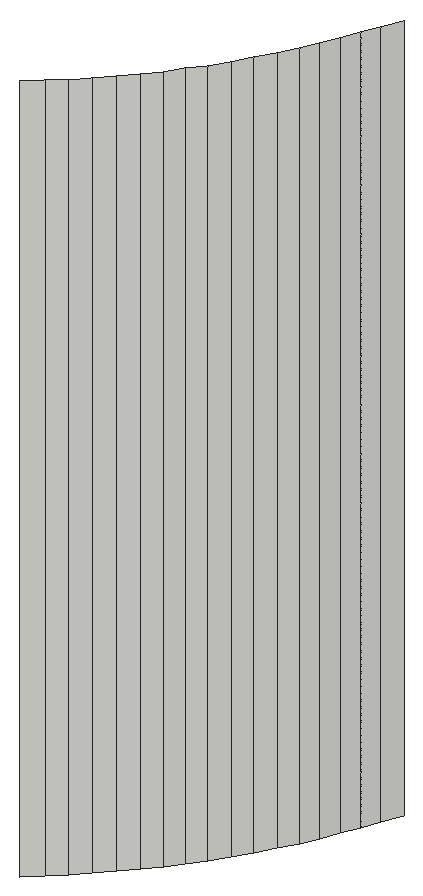
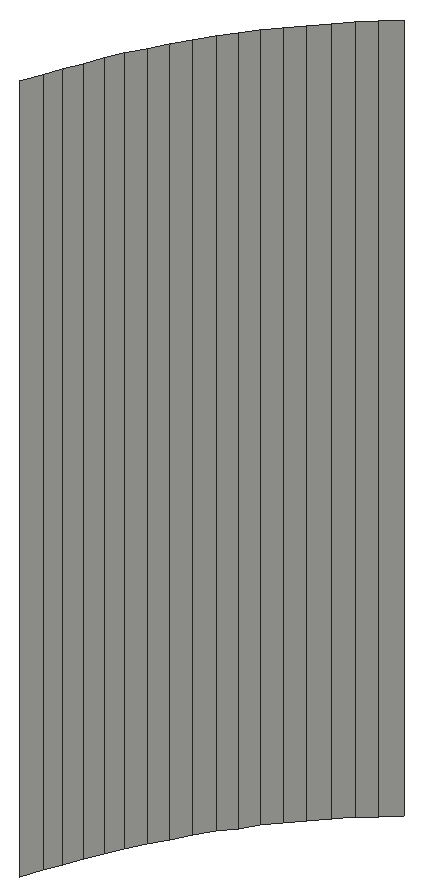
# SketchUp Ruby script. Lengths in inches.
U = 1.inch
M = Sketchup.active_model
def pt(a) = Geom::Point3d.new(a.map { |v| v * U })
def face(e, loops, mat)
  f = e.add_face(loops[0].map { |a| pt(a) })
  loops[1..].each { |l| e.add_face(l.map { |a| pt(a) }).erase! }
  f.material = f.back_material = mat if mat
  f
end
# faces: each face lists its corners as indices into pts; further lists are holes
def faces(e, pts, list, mat = nil) = list.each { |f| face(e, (f[0].is_a?(Array) ? f : [f]).map { |l| l.map { |i| pts[i] } }, mat) }
# xy, xz, yz: faces in a plane at the given z, y or x. An outline is a flat list of corners, or four numbers for a rectangle; further outlines are holes
def ring(l) = l.size == 4 ? [[l[0], l[1]], [l[2], l[1]], [l[2], l[3]], [l[0], l[3]]] : l.each_slice(2).to_a
def flat(e, list, mat, &to3) = list.each { |f| face(e, (f[0].is_a?(Array) ? f : [f]).map { |l| ring(l).map { |u, v| to3.(u, v) } }, mat) }
def xy(e, z, list, mat = nil) = flat(e, list, mat) { |x, y| [x, y, z] }
def xz(e, y, list, mat = nil) = flat(e, list, mat) { |x, z| [x, y, z] }
def yz(e, x, list, mat = nil) = flat(e, list, mat) { |y, z| [x, y, z] }
def lines(e, pts, list) = list.each { |a, b| e.add_line(pt(pts[a]), pt(pts[b])) }
# prism: a flat outline (further loops are holes) pulled along v
def prism(e, loops, v, mat = nil)
  f = face(e, loops, mat); d = Geom::Vector3d.new(v.map { |x| x * U })
  f.pushpull(f.normal.samedirection?(d) ? d.length : -d.length)
end
def box(e, o, s, mat = nil) = prism(e, [[o, [o[0] + s[0], o[1], o[2]], [o[0] + s[0], o[1] + s[1], o[2]], [o[0], o[1] + s[1], o[2]]]], [0, 0, s[2]], mat)
def at(x, y, z, deg = 0) = Geom::Transformation.translation(pt([x, y, z])) * Geom::Transformation.rotation(ORIGIN, Z_AXIS, deg.degrees)
def axes(o, x, y, z) = Geom::Transformation.new([*x, 0, *y, 0, *z, 0, *pt(o).to_a, 1])
def part(name) = M.definitions.add(name)
# library, detail: a bought-in or finely detailed component or shape, given as its bounding box
def library(name, o, s) = part(name).tap { |d| box(d.entities, o, s) }
def detail(e, o, s) = box(e.add_group.entities, o, s)
def put(e, d, t, mat = nil) = e.add_instance(d, t).tap { |i| i.material = mat if mat }
def group(e, t, mat = nil) = e.add_group.tap { |g| g.transformation = t; g.material = mat if mat }.entities
root = M.entities
p = [[88.71,189.18,242],[88.65,189.125,242],[88.65,189.125,245],[88.71,189.18,245],[88.77,189.23,242],[88.77,189.23,245],
  [88.82,189.29,242],[88.82,189.29,245],[88.875,189.35,242],[88.875,189.35,245],[88.93,189.41,242],[88.93,189.41,245],
  [88.98,189.47,242],[88.98,189.47,245],[89.02,189.53,242],[89.02,189.53,245],[89.07,189.59,242],[89.07,189.59,245],
  [89.11,189.66,242],[89.11,189.66,245],[89.15,189.73,242],[89.15,189.73,245],[89.19,189.8,242],[89.19,189.8,245],
  [89.23,189.87,242],[89.23,189.87,245],[89.26,189.9375,242],[89.26,189.9375,245],[89.29,190.01,242],[89.29,190.01,245],
  [89.32,190.08,242],[89.32,190.08,245],[89.35,190.15,242],[89.35,190.15,245],[89.38,190.23,242],[89.38,190.23,245]]
faces(root,p,[[0,1,2,3],[4,0,3,5],[6,4,5,7],[8,6,7,9],[10,8,9,11],[12,10,11,13],[14,12,13,15],[16,14,15,17],
  [18,16,17,19],[20,18,19,21],[22,20,21,23],[24,22,23,25],[26,24,25,27],[28,26,27,29],[30,28,29,31],[32,30,31,33],
  [34,32,33,35]])
